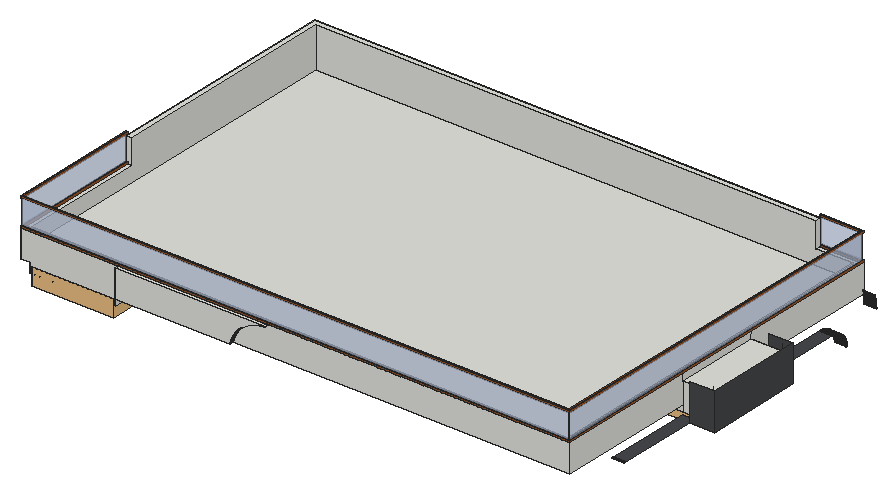
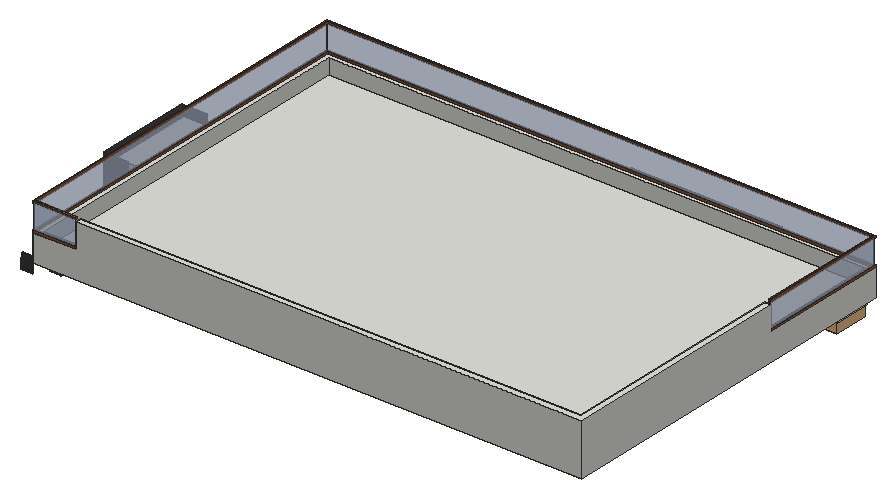
# SketchUp Ruby script. Lengths in inches.
U = 1.inch
M = Sketchup.active_model
def pt(a) = Geom::Point3d.new(a.map { |v| v * U })
def face(e, loops, mat)
  f = e.add_face(loops[0].map { |a| pt(a) })
  loops[1..].each { |l| e.add_face(l.map { |a| pt(a) }).erase! }
  f.material = f.back_material = mat if mat
  f
end
# faces: each face lists its corners as indices into pts; further lists are holes
def faces(e, pts, list, mat = nil) = list.each { |f| face(e, (f[0].is_a?(Array) ? f : [f]).map { |l| l.map { |i| pts[i] } }, mat) }
# xy, xz, yz: faces in a plane at the given z, y or x. An outline is a flat list of corners, or four numbers for a rectangle; further outlines are holes
def ring(l) = l.size == 4 ? [[l[0], l[1]], [l[2], l[1]], [l[2], l[3]], [l[0], l[3]]] : l.each_slice(2).to_a
def flat(e, list, mat, &to3) = list.each { |f| face(e, (f[0].is_a?(Array) ? f : [f]).map { |l| ring(l).map { |u, v| to3.(u, v) } }, mat) }
def xy(e, z, list, mat = nil) = flat(e, list, mat) { |x, y| [x, y, z] }
def xz(e, y, list, mat = nil) = flat(e, list, mat) { |x, z| [x, y, z] }
def yz(e, x, list, mat = nil) = flat(e, list, mat) { |y, z| [x, y, z] }
def lines(e, pts, list) = list.each { |a, b| e.add_line(pt(pts[a]), pt(pts[b])) }
# prism: a flat outline (further loops are holes) pulled along v
def prism(e, loops, v, mat = nil)
  f = face(e, loops, mat); d = Geom::Vector3d.new(v.map { |x| x * U })
  f.pushpull(f.normal.samedirection?(d) ? d.length : -d.length)
end
def box(e, o, s, mat = nil) = prism(e, [[o, [o[0] + s[0], o[1], o[2]], [o[0] + s[0], o[1] + s[1], o[2]], [o[0], o[1] + s[1], o[2]]]], [0, 0, s[2]], mat)
def at(x, y, z, deg = 0) = Geom::Transformation.translation(pt([x, y, z])) * Geom::Transformation.rotation(ORIGIN, Z_AXIS, deg.degrees)
def axes(o, x, y, z) = Geom::Transformation.new([*x, 0, *y, 0, *z, 0, *pt(o).to_a, 1])
def part(name) = M.definitions.add(name)
# library, detail: a bought-in or finely detailed component or shape, given as its bounding box
def library(name, o, s) = part(name).tap { |d| box(d.entities, o, s) }
def detail(e, o, s) = box(e.add_group.entities, o, s)
def put(e, d, t, mat = nil) = e.add_instance(d, t).tap { |i| i.material = mat if mat }
def group(e, t, mat = nil) = e.add_group.tap { |g| g.transformation = t; g.material = mat if mat }.entities
root = M.entities
M.materials.add("1432 AP 8245 TAR ROAD").color = [71, 72, 75]
M.materials.add("[Translucent Glass Blue]").color = [195, 208, 233]
M.materials["[Translucent Glass Blue]"].alpha = 0.5
M.materials.add("[Wood Cherry Original]").color = [152, 86, 42]
c1 = library("Group\#32",[0,0,-17.09],[62,80,17.09])
xy(root,560.79,[[573,160.9,585,161.13],[573,161.13,585,161.37],[573,161.37,573,245.37,603,245.37,603,329.37,573,329.37,573,413.37,585,413.37,585,335.37,609,335.37,609,239.37,585,239.37,585,161.37],[573,413.37,585,413.61],[573,413.61,585,413.84]],"1432 AP 8245 TAR ROAD")
xz(root,239.37,[[585,560.79,609,596.79]],"1432 AP 8245 TAR ROAD")
xz(root,335.37,[[585,560.79,609,596.79]],"1432 AP 8245 TAR ROAD")
xz(root,431.36,[[573,543.26,585,543.5]],"1432 AP 8245 TAR ROAD")
xz(root,431.37,[[573,542.79,585,543.03]],"1432 AP 8245 TAR ROAD")
xz(root,467.37,[[573,560.79,585,561.07],[573,561.07,585,561.36]],"1432 AP 8245 TAR ROAD")
yz(root,609,[[239.37,560.79,335.37,596.79]],"1432 AP 8245 TAR ROAD")
p = [[573,431.36,543.26],[573,431.37,543.03],[585,431.37,543.03],[585,431.36,543.26],[573,431.35,543.73],[573,431.36,543.5],
  [585,431.36,543.5],[585,431.35,543.73],[573,431.33,543.97],[585,431.33,543.97],[573,431.3125,544.2],[585,431.3125,544.2],
  [573,431.29,544.4375],[585,431.29,544.4375],[573,431.27,544.67],[585,431.27,544.67],[573,431.25,544.91],[585,431.25,544.91],
  [573,431.22,545.14],[585,431.22,545.14],[573,431.18,545.375],[585,431.18,545.375],[573,431.15,545.61],[585,431.15,545.61],
  [573,431.11,545.84],[585,431.11,545.84],[573,431.07,546.07],[585,431.07,546.07],[573,431.02,546.3],[585,431.02,546.3],
  [573,430.98,546.53],[585,430.98,546.53],[573,430.93,546.76],[585,430.93,546.76],[573,430.87,546.99],[585,430.87,546.99],
  [573,430.82,547.22],[585,430.82,547.22],[573,430.76,547.45],[585,430.76,547.45],[573,430.69,547.68],[585,430.69,547.68],
  [573,430.63,547.9],[585,430.63,547.9],[573,430.56,548.13],[585,430.56,548.13],[573,430.49,548.35],[585,430.49,548.35],
  [573,430.41,548.58],[585,430.41,548.58],[573,430.34,548.8],[585,430.34,548.8],[573,430.26,549.02],[585,430.26,549.02],
  [573,430.17,549.24],[585,430.17,549.24],[573,430.09,549.46],[585,430.09,549.46],[573,430,549.68],[585,430,549.68],
  [573,429.91,549.9],[585,429.91,549.9],[573,429.8125,550.11],[585,429.8125,550.11],[573,429.72,550.33],[585,429.72,550.33],
  [573,429.62,550.54],[585,429.62,550.54],[573,429.51,550.75],[585,429.51,550.75],[573,429.41,550.96],[585,429.41,550.96],
  [573,429.3,551.17],[585,429.3,551.17],[573,429.1875,551.38],[585,429.1875,551.38],[573,429.07,551.59],[585,429.07,551.59],
  [573,428.96,551.79],[585,428.96,551.79],[573,428.84,552],[585,428.84,552],[573,428.72,552.2],[585,428.72,552.2],
  [573,428.59,552.4],[585,428.59,552.4],[573,428.47,552.6],[585,428.47,552.6],[573,428.34,552.79],[585,428.34,552.79],
  [573,428.2,552.99],[585,428.2,552.99],[573,428.07,553.18],[585,428.07,553.18],[573,427.93,553.37],[585,427.93,553.37],
  [573,427.79,553.5625],[585,427.79,553.5625],[573,427.65,553.75],[585,427.65,553.75],[573,427.51,553.9375],[585,427.51,553.9375],
  [573,427.36,554.12],[585,427.36,554.12],[573,427.21,554.3],[585,427.21,554.3],[573,427.06,554.48],[585,427.06,554.48],
  [573,426.9,554.66],[585,426.9,554.66],[573,426.75,554.84],[585,426.75,554.84],[573,426.59,555.01],[585,426.59,555.01],
  [573,426.43,555.18],[585,426.43,555.18],[573,426.26,555.35],[585,426.26,555.35],[573,426.1,555.52],[585,426.1,555.52],
  [573,425.93,555.69],[585,425.93,555.69],[573,425.76,555.85],[585,425.76,555.85],[573,425.59,556.01],[585,425.59,556.01],
  [573,425.41,556.17],[585,425.41,556.17],[573,425.24,556.33],[585,425.24,556.33],[573,425.06,556.48],[585,425.06,556.48],
  [573,424.88,556.63],[585,424.88,556.63],[573,424.7,556.78],[585,424.7,556.78],[573,424.51,556.93],[585,424.51,556.93],
  [573,424.33,557.07],[585,424.33,557.07],[573,424.14,557.21],[585,424.14,557.21],[573,423.95,557.35],[585,423.95,557.35],
  [573,423.76,557.49],[585,423.76,557.49],[573,423.57,557.625],[585,423.57,557.625],[573,423.37,557.76],[585,423.37,557.76],
  [573,423.17,557.89],[585,423.17,557.89],[573,422.97,558.02],[585,422.97,558.02],[573,422.77,558.14],[585,422.77,558.14],
  [573,422.57,558.26],[585,422.57,558.26],[573,422.37,558.38],[585,422.37,558.38],[573,422.17,558.5],[585,422.17,558.5],
  [573,421.96,558.61],[585,421.96,558.61],[573,421.75,558.72],[585,421.75,558.72],[573,421.54,558.83],[585,421.54,558.83],
  [573,421.33,558.9375],[585,421.33,558.9375],[573,421.12,559.04],[585,421.12,559.04],[573,420.91,559.14],[585,420.91,559.14],
  [573,420.69,559.24],[585,420.69,559.24],[573,420.48,559.33],[585,420.48,559.33],[573,420.26,559.42],[585,420.26,559.42],
  [573,420.04,559.51],[585,420.04,559.51],[573,419.82,559.6],[585,419.82,559.6],[573,419.6,559.68],[585,419.6,559.68],
  [573,419.38,559.76],[585,419.38,559.76],[573,418.93,559.91],[573,419.16,559.84],[585,419.16,559.84],[585,418.93,559.91],
  [573,418.71,559.98],[585,418.71,559.98],[573,418.48,560.05],[585,418.48,560.05],[573,418.03,560.18],[573,418.26,560.12],
  [585,418.26,560.12],[585,418.03,560.18],[573,417.57,560.29],[573,417.8,560.24],[585,417.8,560.24],[585,417.57,560.29],
  [573,417.11,560.4],[573,417.34,560.35],[585,417.34,560.35],[585,417.11,560.4],[573,416.65,560.49],[573,416.88,560.45],
  [585,416.88,560.45],[585,416.65,560.49],[573,416.1875,560.57],[573,416.42,560.53],[585,416.42,560.53],[585,416.1875,560.57],
  [573,415.49,560.67],[573,415.72,560.64],[585,415.72,560.64],[585,415.49,560.67],[573,415.95,560.61],[585,415.95,560.61],
  [573,159.25,560.67],[573,159.49,560.69],[585,159.49,560.69],[585,159.25,560.67],[573,159.72,560.72],[585,159.72,560.72],
  [573,159.96,560.74],[585,159.96,560.74],[573,160.19,560.75],[585,160.19,560.75],[573,414.55,560.75],[573,414.78,560.74],
  [585,414.78,560.74],[585,414.55,560.75],[573,415.02,560.72],[585,415.02,560.72],[573,415.25,560.69],[585,415.25,560.69],
  [573,160.43,560.77],[585,160.43,560.77],[573,160.66,560.78],[585,160.66,560.78],[573,160.9,560.79],[585,160.9,560.79],
  [573,413.84,560.79],[573,414.08,560.78],[585,414.08,560.78],[585,413.84,560.79],[573,414.3125,560.77],[585,414.3125,560.77],
  [573,467.37,561.36],[573,467.36,561.64],[585,467.36,561.64],[585,467.37,561.36],[573,467.35,561.92],[585,467.35,561.92],
  [573,467.34,562.21],[585,467.34,562.21],[573,467.33,562.49],[585,467.33,562.49],[573,467.32,562.77],[585,467.32,562.77],
  [573,467.3,563.05],[585,467.3,563.05],[573,467.28,563.33],[585,467.28,563.33],[573,467.26,563.62],[585,467.26,563.62],
  [573,467.24,563.9],[585,467.24,563.9],[573,467.21,564.18],[585,467.21,564.18],[573,467.18,564.46],[585,467.18,564.46],
  [573,467.15,564.74],[585,467.15,564.74],[573,467.12,565.02],[585,467.12,565.02],[573,467.09,565.3],[585,467.09,565.3],
  [573,467.05,565.58],[585,467.05,565.58],[573,467.01,565.86],[585,467.01,565.86],[573,466.97,566.14],[585,466.97,566.14],
  [573,466.93,566.42],[585,466.93,566.42],[573,466.88,566.7],[585,466.88,566.7],[573,466.83,566.98],[585,466.83,566.98],
  [573,466.78,567.26],[585,466.78,567.26],[573,466.73,567.54],[585,466.73,567.54],[573,466.68,567.82],[585,466.68,567.82],
  [573,466.62,568.09],[585,466.62,568.09],[573,466.5625,568.37],[585,466.5625,568.37],[573,466.5,568.65],[585,466.5,568.65],
  [573,466.44,568.92],[585,466.44,568.92],[573,466.375,569.2],[585,466.375,569.2],[573,466.31,569.47],[585,466.31,569.47],
  [573,466.24,569.74],[585,466.24,569.74],[573,466.17,570.02],[585,466.17,570.02],[573,466.09,570.29],[585,466.09,570.29],
  [573,466.02,570.5625],[585,466.02,570.5625],[573,465.94,570.84],[585,465.94,570.84],[573,465.86,571.11],[585,465.86,571.11],
  [573,465.78,571.38],[585,465.78,571.38],[573,465.69,571.65],[585,465.69,571.65],[573,465.61,571.92],[585,465.61,571.92],
  [573,465.52,572.19],[585,465.52,572.19],[573,465.43,572.45],[585,465.43,572.45],[573,465.34,572.72],[585,465.34,572.72],
  [573,465.24,572.99],[585,465.24,572.99],[573,465.14,573.25],[585,465.14,573.25],[573,465.05,573.52],[585,465.05,573.52],
  [573,464.94,573.78],[585,464.94,573.78],[573,464.84,574.04],[585,464.84,574.04],[573,464.74,574.31],[585,464.74,574.31],
  [603,245.37,596.79],[603,245.37,560.79],[603,329.37,596.79],[603,329.37,560.79]]
faces(root,p,[[0,1,2,3],[4,5,6,7],[8,4,7,9],[10,8,9,11],[12,10,11,13],[14,12,13,15],[16,14,15,17],[18,16,17,19],
  [20,18,19,21],[22,20,21,23],[24,22,23,25],[26,24,25,27],[28,26,27,29],[30,28,29,31],[32,30,31,33],[34,32,33,35],
  [36,34,35,37],[38,36,37,39],[40,38,39,41],[42,40,41,43],[44,42,43,45],[46,44,45,47],[48,46,47,49],[50,48,49,51],
  [52,50,51,53],[54,52,53,55],[56,54,55,57],[58,56,57,59],[60,58,59,61],[62,60,61,63],[64,62,63,65],[66,64,65,67],
  [68,66,67,69],[70,68,69,71],[72,70,71,73],[74,72,73,75],[76,74,75,77],[78,76,77,79],[80,78,79,81],[82,80,81,83],
  [84,82,83,85],[86,84,85,87],[88,86,87,89],[90,88,89,91],[92,90,91,93],[94,92,93,95],[96,94,95,97],[98,96,97,99],
  [100,98,99,101],[102,100,101,103],[104,102,103,105],[106,104,105,107],[108,106,107,109],[110,108,109,111],[112,110,111,113],[114,112,113,115],
  [116,114,115,117],[118,116,117,119],[120,118,119,121],[122,120,121,123],[124,122,123,125],[126,124,125,127],[128,126,127,129],[130,128,129,131],
  [132,130,131,133],[134,132,133,135],[136,134,135,137],[138,136,137,139],[140,138,139,141],[142,140,141,143],[144,142,143,145],[146,144,145,147],
  [148,146,147,149],[150,148,149,151],[152,150,151,153],[154,152,153,155],[156,154,155,157],[158,156,157,159],[160,158,159,161],[162,160,161,163],
  [164,162,163,165],[166,164,165,167],[168,166,167,169],[170,168,169,171],[172,170,171,173],[174,172,173,175],[176,174,175,177],[178,176,177,179],
  [180,178,179,181],[182,180,181,183],[184,182,183,185],[186,184,185,187],[188,189,190,191],[189,186,187,190],[192,188,191,193],[194,192,193,195],
  [196,197,198,199],[197,194,195,198],[200,201,202,203],[201,196,199,202],[204,205,206,207],[205,200,203,206],[208,209,210,211],[209,204,207,210],
  [212,213,214,215],[213,208,211,214],[216,217,218,219],[217,220,221,218],[220,212,215,221],[222,223,224,225],[223,226,227,224],[226,228,229,227],
  [228,230,231,229],[232,233,234,235],[233,236,237,234],[236,238,239,237],[238,216,219,239],[230,240,241,231],[240,242,243,241],[242,244,245,243],
  [246,247,248,249],[247,250,251,248],[250,232,235,251],[252,253,254,255],[253,256,257,254],[256,258,259,257],[258,260,261,259],[260,262,263,261],
  [262,264,265,263],[264,266,267,265],[266,268,269,267],[268,270,271,269],[270,272,273,271],[272,274,275,273],[274,276,277,275],[276,278,279,277],
  [278,280,281,279],[280,282,283,281],[282,284,285,283],[284,286,287,285],[286,288,289,287],[288,290,291,289],[290,292,293,291],[292,294,295,293],
  [294,296,297,295],[296,298,299,297],[298,300,301,299],[300,302,303,301],[302,304,305,303],[304,306,307,305],[306,308,309,307],[308,310,311,309],
  [310,312,313,311],[312,314,315,313],[314,316,317,315],[316,318,319,317],[318,320,321,319],[320,322,323,321],[322,324,325,323],[324,326,327,325],
  [326,328,329,327],[328,330,331,329],[330,332,333,331],[332,334,335,333],[334,336,337,335],[336,338,339,337],[338,340,341,339],[340,342,343,341],
  [342,344,345,343],[344,346,347,345]],"1432 AP 8245 TAR ROAD")
lines(root,p,[[348,349],[350,351]])
g1 = group(root,at(45,116.37,569.79))
xy(g1,-9,[[[0,-8.9375,84,27],[2,-6.9375,82,25]]])
xy(g1,-6,[[[492,129,558,213],[494,131,556,211]]])
xy(g1,-3,[[2,-6.9375,82,25]])
xy(g1,0,[[87,-13,87,-8.9375,84,-8.9375,84,27,0,27,0,-8.9375,-9,-8.9375,-9,351,528,351,528,213,492,213,492,129,528,129,528,-9,199.14,-9,199.14,-13]])
xy(g1,2,[[494,131,556,211]])
xy(g1,12,[[-3,-3,522,345]])
xy(g1,21,[[528,129,558,213]])
xy(g1,27,[[87,-13,234,-13,234,-9,528,-9,528,351,486,351,486,345,522,345,522,-3,-3,-3,-3,120.0625,-9,120.0625,-9,-8.9375,87,-8.9375],[233.6,-13,234,-9]])
xy(g1,51,[[-9,120.0625,-3,120.0625,-3,345,486,345,486,351,-9,351]])
xz(g1,-13,[[87,0,199.14,0,199.25,0.38,199.35,0.76,199.46,1.14,199.58,1.52,199.69,1.9,199.82,2.27,199.94,2.65,200.07,3.02,200.49,4.13,200.64,4.5,200.79,4.86,200.94,5.23,201.1,5.59,201.27,5.95,201.43,6.31,201.6,6.66,201.78,7.02,202.14,7.72,202.52,8.42,202.71,8.76,203.11,9.44,203.3125,9.78,203.52,10.12,203.73,10.45,204.17,11.11,204.39,11.43,204.62,11.76,205.08,12.4,205.32,12.71,205.56,13.03,205.8,13.34,206.05,13.65,206.3,13.95,206.56,14.26,206.8125,14.56,207.07,14.85,207.34,15.15,207.61,15.4375,207.875,15.73,208.15,16.01,208.99,16.85,209.27,17.12,209.5625,17.39,209.85,17.66,210.75,18.44,211.35,18.94,211.97,19.44,212.29,19.68,212.6,19.91,212.92,20.15,213.24,20.375,213.57,20.6,213.9,20.82,214.22,21.04,214.56,21.26,215.22,21.68,215.5625,21.88,215.9,22.09,216.25,22.28,216.59,22.48,216.9375,22.67,217.29,22.85,218.34,23.39,218.7,23.56,219.06,23.72,219.42,23.89,219.78,24.04,220.14,24.2,220.88,24.5,221.62,24.78,222.36,25.04,222.74,25.17,223.11,25.29,223.49,25.41,224.25,25.63,224.625,25.74,225.01,25.84,225.39,25.9375,225.78,26.03,226.16,26.12,226.55,26.2,226.93,26.28,227.32,26.36,228.1,26.5,228.49,26.5625,228.88,26.62,229.27,26.68,229.66,26.73,230.06,26.77,230.45,26.82,230.84,26.85,231.24,26.89,231.63,26.92,232.03,26.94,232.81,26.98,233.21,26.99,233.6,27,234,27,87,27]])
xz(g1,-9,[[199.14,0,528,0,528,27,233.6,27,233.21,26.99,232.81,26.98,232.03,26.94,231.63,26.92,231.24,26.89,230.84,26.85,230.45,26.82,230.06,26.77,229.66,26.73,229.27,26.68,228.88,26.62,228.49,26.5625,228.1,26.5,227.32,26.36,226.93,26.28,226.55,26.2,226.16,26.12,225.78,26.03,225.39,25.9375,225.01,25.84,224.625,25.74,224.25,25.63,223.49,25.41,223.11,25.29,222.74,25.17,222.36,25.04,221.62,24.78,220.88,24.5,220.14,24.2,219.78,24.04,219.42,23.89,219.06,23.72,218.7,23.56,218.34,23.39,217.29,22.85,216.9375,22.67,216.59,22.48,216.25,22.28,215.9,22.09,215.5625,21.88,215.22,21.68,214.56,21.26,214.22,21.04,213.9,20.82,213.57,20.6,213.24,20.375,212.92,20.15,212.6,19.91,212.29,19.68,211.97,19.44,211.35,18.94,210.75,18.44,209.85,17.66,209.5625,17.39,209.27,17.12,208.99,16.85,208.15,16.01,207.875,15.73,207.61,15.4375,207.34,15.15,207.07,14.85,206.8125,14.56,206.56,14.26,206.3,13.95,206.05,13.65,205.8,13.34,205.56,13.03,205.32,12.71,205.08,12.4,204.62,11.76,204.39,11.43,204.17,11.11,203.73,10.45,203.52,10.12,203.3125,9.78,203.11,9.44,202.71,8.76,202.52,8.42,202.14,7.72,201.78,7.02,201.6,6.66,201.43,6.31,201.27,5.95,201.1,5.59,200.94,5.23,200.79,4.86,200.64,4.5,200.49,4.13,200.07,3.02,199.94,2.65,199.82,2.27,199.69,1.9,199.58,1.52,199.46,1.14,199.35,0.76,199.25,0.38]])
xz(g1,-8.9375,[[0,-9,84,-9,84,0,87,0,87,27,-9,27,-9,0,0,0]])
xz(g1,-6.9375,[[2,-9,82,-3]])
xz(g1,-3,[[-3,12,522,27]])
xz(g1,25,[[2,-9,82,-3]])
xz(g1,27,[[0,-9,84,0]])
xz(g1,120.0625,[[-9,27,-3,51]])
xz(g1,129,[[492,-6,528,0],[528,-6,558,21]])
xz(g1,131,[[494,-6,528,2],[528,-6,556,2]])
xz(g1,211,[[494,-6,528,2],[528,-6,556,2]])
xz(g1,213,[[492,-6,528,0],[528,-6,558,21]])
xz(g1,345,[[-3,12,522,12,522,27,486,27,486,51,-3,51]])
xz(g1,351,[[-9,0,-9,51,486,51,486,27,528,27,528,0]])
yz(g1,-9,[[-8.9375,0,-8.9375,27,120.0625,27,120.0625,51,351,51,351,0]])
yz(g1,-3,[[-3,12,345,12,345,51,120.0625,51,120.0625,27,-3,27]])
yz(g1,0,[[-8.9375,-9,27,0]])
yz(g1,2,[[-6.9375,-9,25,-3]])
yz(g1,82,[[-6.9375,-9,25,-3]])
yz(g1,84,[[-8.9375,-9,27,0]])
yz(g1,87,[[-13,0,-8.9375,27]])
yz(g1,486,[[345,27,351,51]])
yz(g1,492,[[129,-6,213,0]])
yz(g1,494,[[131,-6,211,2]])
yz(g1,522,[[-3,12,345,27]])
yz(g1,528,[[-9,0,129,27],[213,0,351,27],[129,21,213,27]])
yz(g1,556,[[131,-6,211,2]])
yz(g1,558,[[129,-6,213,21]])
p = [[199.25,-13,0.38],[199.14,-13,0],[199.14,-9,0],[199.25,-9,0.38],[199.35,-13,0.76],[199.35,-9,0.76],
  [199.46,-13,1.14],[199.46,-9,1.14],[199.58,-13,1.52],[199.58,-9,1.52],[199.69,-13,1.9],[199.69,-9,1.9],
  [199.82,-13,2.27],[199.82,-9,2.27],[199.94,-13,2.65],[199.94,-9,2.65],[200.07,-13,3.02],[200.07,-9,3.02],
  [200.21,-13,3.39],[200.21,-9,3.39],[200.35,-13,3.76],[200.35,-9,3.76],[200.49,-13,4.13],[200.49,-9,4.13],
  [200.64,-13,4.5],[200.64,-9,4.5],[200.79,-13,4.86],[200.79,-9,4.86],[200.94,-13,5.23],[200.94,-9,5.23],
  [201.1,-13,5.59],[201.1,-9,5.59],[201.27,-13,5.95],[201.27,-9,5.95],[201.43,-13,6.31],[201.43,-9,6.31],
  [201.6,-13,6.66],[201.6,-9,6.66],[201.78,-13,7.02],[201.78,-9,7.02],[201.96,-13,7.37],[201.96,-9,7.37],
  [202.14,-13,7.72],[202.14,-9,7.72],[202.33,-13,8.07],[202.33,-9,8.07],[202.52,-13,8.42],[202.52,-9,8.42],
  [202.71,-13,8.76],[202.71,-9,8.76],[202.91,-13,9.1],[202.91,-9,9.1],[203.11,-13,9.44],[203.11,-9,9.44],
  [203.3125,-13,9.78],[203.3125,-9,9.78],[203.52,-13,10.12],[203.52,-9,10.12],[203.73,-13,10.45],[203.73,-9,10.45],
  [203.95,-13,10.78],[203.95,-9,10.78],[204.17,-13,11.11],[204.17,-9,11.11],[204.39,-13,11.43],[204.39,-9,11.43],
  [204.62,-13,11.76],[204.62,-9,11.76],[204.85,-13,12.08],[204.85,-9,12.08],[205.08,-13,12.4],[205.08,-9,12.4],
  [205.32,-13,12.71],[205.32,-9,12.71],[205.56,-13,13.03],[205.56,-9,13.03],[205.8,-13,13.34],[205.8,-9,13.34],
  [206.05,-13,13.65],[206.05,-9,13.65],[206.3,-13,13.95],[206.3,-9,13.95],[206.56,-13,14.26],[206.56,-9,14.26],
  [206.8125,-13,14.56],[206.8125,-9,14.56],[207.07,-13,14.85],[207.07,-9,14.85],[207.34,-13,15.15],[207.34,-9,15.15],
  [207.61,-13,15.4375],[207.61,-9,15.4375],[207.875,-13,15.73],[207.875,-9,15.73],[208.15,-13,16.01],[208.15,-9,16.01],
  [208.43,-13,16.29],[208.43,-9,16.29],[208.71,-13,16.57],[208.71,-9,16.57],[208.99,-13,16.85],[208.99,-9,16.85],
  [209.27,-13,17.12],[209.27,-9,17.12],[209.5625,-13,17.39],[209.5625,-9,17.39],[209.85,-13,17.66],[209.85,-9,17.66],
  [210.15,-13,17.92],[210.15,-9,17.92],[210.45,-13,18.18],[210.45,-9,18.18],[210.75,-13,18.44],[210.75,-9,18.44],
  [211.05,-13,18.69],[211.05,-9,18.69],[211.35,-13,18.94],[211.35,-9,18.94],[211.66,-13,19.19],[211.66,-9,19.19],
  [211.97,-13,19.44],[211.97,-9,19.44],[212.29,-13,19.68],[212.29,-9,19.68],[212.6,-13,19.91],[212.6,-9,19.91],
  [212.92,-13,20.15],[212.92,-9,20.15],[213.24,-13,20.375],[213.24,-9,20.375],[213.57,-13,20.6],[213.57,-9,20.6],
  [213.9,-13,20.82],[213.9,-9,20.82],[214.22,-13,21.04],[214.22,-9,21.04],[214.56,-13,21.26],[214.56,-9,21.26],
  [214.89,-13,21.47],[214.89,-9,21.47],[215.22,-13,21.68],[215.22,-9,21.68],[215.5625,-13,21.88],[215.5625,-9,21.88],
  [215.9,-13,22.09],[215.9,-9,22.09],[216.25,-13,22.28],[216.25,-9,22.28],[216.59,-13,22.48],[216.59,-9,22.48],
  [216.9375,-13,22.67],[216.9375,-9,22.67],[217.29,-13,22.85],[217.29,-9,22.85],[217.64,-13,23.03],[217.64,-9,23.03],
  [217.99,-13,23.21],[217.99,-9,23.21],[218.34,-13,23.39],[218.34,-9,23.39],[218.7,-13,23.56],[218.7,-9,23.56],
  [219.06,-13,23.72],[219.06,-9,23.72],[219.42,-13,23.89],[219.42,-9,23.89],[219.78,-13,24.04],[219.78,-9,24.04],
  [220.14,-13,24.2],[220.14,-9,24.2],[220.51,-13,24.35],[220.51,-9,24.35],[220.88,-13,24.5],[220.88,-9,24.5],
  [221.25,-13,24.64],[221.25,-9,24.64],[221.62,-13,24.78],[221.62,-9,24.78],[221.99,-13,24.91],[221.99,-9,24.91],
  [222.36,-13,25.04],[222.36,-9,25.04],[222.74,-13,25.17],[222.74,-9,25.17],[223.11,-13,25.29],[223.11,-9,25.29],
  [223.49,-13,25.41],[223.49,-9,25.41],[223.87,-13,25.52],[223.87,-9,25.52],[224.25,-13,25.63],[224.25,-9,25.63],
  [224.625,-13,25.74],[224.625,-9,25.74],[225.01,-13,25.84],[225.01,-9,25.84],[225.39,-13,25.9375],[225.39,-9,25.9375],
  [225.78,-13,26.03],[225.78,-9,26.03],[226.16,-13,26.12],[226.16,-9,26.12],[226.55,-13,26.2],[226.55,-9,26.2],
  [226.93,-13,26.28],[226.93,-9,26.28],[227.32,-13,26.36],[227.32,-9,26.36],[227.71,-13,26.43],[227.71,-9,26.43],
  [228.1,-13,26.5],[228.1,-9,26.5],[228.49,-13,26.5625],[228.49,-9,26.5625],[228.88,-13,26.62],[228.88,-9,26.62],
  [229.27,-13,26.68],[229.27,-9,26.68],[229.66,-13,26.73],[229.66,-9,26.73],[230.06,-13,26.77],[230.06,-9,26.77],
  [230.45,-13,26.82],[230.45,-9,26.82],[230.84,-13,26.85],[230.84,-9,26.85],[231.24,-13,26.89],[231.24,-9,26.89],
  [231.63,-13,26.92],[231.63,-9,26.92],[232.03,-13,26.94],[232.03,-9,26.94],[232.42,-13,26.96],[232.42,-9,26.96],
  [232.81,-13,26.98],[232.81,-9,26.98],[233.21,-13,26.99],[233.21,-9,26.99],[233.6,-13,27],[233.6,-9,27],
  [199.28,-9,0.5],[199.36,-9,0.8],[199.45,-9,1.1],[199.54,-9,1.4],[199.63,-9,1.7],[199.72,-9,2],
  [199.82,-9,2.3],[199.92,-9,2.59],[200.02,-9,2.89],[200.125,-9,3.18],[200.23,-9,3.48],[200.34,-9,3.77],
  [200.45,-9,4.0625],[200.57,-9,4.35],[200.6875,-9,4.64],[200.81,-9,4.93],[200.93,-9,5.22],[201.05,-9,5.51],
  [201.18,-9,5.79],[201.31,-9,6.08],[201.44,-9,6.36],[201.58,-9,6.64],[201.71,-9,6.93],[201.85,-9,7.21],
  [202,-9,7.48],[202.14,-9,7.76],[202.29,-9,8.04],[202.4375,-9,8.3125],[202.59,-9,8.59],[202.74,-9,8.86],
  [202.9,-9,9.13],[203.06,-9,9.4],[203.22,-9,9.67],[203.38,-9,9.94],[203.55,-9,10.2],[203.72,-9,10.46],
  [203.89,-9,10.73],[204.06,-9,10.99],[204.23,-9,11.25],[204.41,-9,11.51],[204.59,-9,11.76],[204.77,-9,12.02],
  [204.96,-9,12.27],[205.14,-9,12.52],[205.33,-9,12.77],[205.52,-9,13.02],[205.71,-9,13.27],[205.91,-9,13.51],
  [206.1,-9,13.76],[206.3,-9,14],[206.5,-9,14.24],[206.71,-9,14.47],[206.91,-9,14.71],[207.12,-9,14.95],
  [207.33,-9,15.18],[207.54,-9,15.41],[207.75,-9,15.64],[207.97,-9,15.87],[208.18,-9,16.09],[208.4,-9,16.3125],
  [208.625,-9,16.54],[208.85,-9,16.76],[209.07,-9,16.97],[209.3,-9,17.1875],[209.53,-9,17.4],[209.76,-9,17.61],
  [209.99,-9,17.82],[210.22,-9,18.03],[210.46,-9,18.24],[210.7,-9,18.44],[210.9375,-9,18.64],[211.18,-9,18.84],
  [211.42,-9,19.04],[211.67,-9,19.23],[211.91,-9,19.43],[212.16,-9,19.62],[212.41,-9,19.81],[212.66,-9,19.99],
  [212.91,-9,20.18],[213.17,-9,20.36],[213.42,-9,20.54],[213.68,-9,20.72],[213.94,-9,20.89],[214.2,-9,21.07],
  [214.46,-9,21.24],[214.73,-9,21.41],[214.99,-9,21.57],[215.26,-9,21.74],[215.53,-9,21.9],[215.79,-9,22.06],
  [216.07,-9,22.21],[216.34,-9,22.37],[216.61,-9,22.52],[216.89,-9,22.67],[217.16,-9,22.82],[217.4375,-9,22.96],
  [217.72,-9,23.11],[218,-9,23.25],[218.28,-9,23.39],[218.56,-9,23.52],[218.84,-9,23.65],[219.13,-9,23.78],
  [219.41,-9,23.91],[219.7,-9,24.04],[219.99,-9,24.16],[220.28,-9,24.28],[220.57,-9,24.4],[220.86,-9,24.51],
  [221.15,-9,24.63],[221.44,-9,24.74],[221.73,-9,24.85],[222.03,-9,24.95],[222.32,-9,25.05],[222.62,-9,25.15],
  [222.92,-9,25.25],[223.22,-9,25.35],[223.52,-9,25.4375],[223.82,-9,25.53],[224.12,-9,25.62],[224.42,-9,25.7],
  [224.72,-9,25.78],[225.02,-9,25.86],[225.32,-9,25.9375],[225.63,-9,26.01],[225.93,-9,26.08],[226.24,-9,26.15],
  [226.54,-9,26.22],[226.85,-9,26.28],[227.16,-9,26.34],[227.47,-9,26.4],[227.77,-9,26.46],[228.08,-9,26.51],
  [228.39,-9,26.56],[228.7,-9,26.61],[229.01,-9,26.65],[229.32,-9,26.69],[229.63,-9,26.73],[229.94,-9,26.77],
  [230.25,-9,26.8],[230.5625,-9,26.84],[230.875,-9,26.86],[231.1875,-9,26.89],[231.5,-9,26.91],[231.8125,-9,26.93],
  [232.125,-9,26.95],[232.4375,-9,26.97],[232.75,-9,26.98],[233.0625,-9,26.99],[233.375,-9,26.99],[233.6875,-9,27],
  [234,-9,27]]
faces(g1,p,[[0,1,2,3],[4,0,3,5],[6,4,5,7],[8,6,7,9],[10,8,9,11],[12,10,11,13],[14,12,13,15],[16,14,15,17],
  [18,16,17,19],[20,18,19,21],[22,20,21,23],[24,22,23,25],[26,24,25,27],[28,26,27,29],[30,28,29,31],[32,30,31,33],
  [34,32,33,35],[36,34,35,37],[38,36,37,39],[40,38,39,41],[42,40,41,43],[44,42,43,45],[46,44,45,47],[48,46,47,49],
  [50,48,49,51],[52,50,51,53],[54,52,53,55],[56,54,55,57],[58,56,57,59],[60,58,59,61],[62,60,61,63],[64,62,63,65],
  [66,64,65,67],[68,66,67,69],[70,68,69,71],[72,70,71,73],[74,72,73,75],[76,74,75,77],[78,76,77,79],[80,78,79,81],
  [82,80,81,83],[84,82,83,85],[86,84,85,87],[88,86,87,89],[90,88,89,91],[92,90,91,93],[94,92,93,95],[96,94,95,97],
  [98,96,97,99],[100,98,99,101],[102,100,101,103],[104,102,103,105],[106,104,105,107],[108,106,107,109],[110,108,109,111],[112,110,111,113],
  [114,112,113,115],[116,114,115,117],[118,116,117,119],[120,118,119,121],[122,120,121,123],[124,122,123,125],[126,124,125,127],[128,126,127,129],
  [130,128,129,131],[132,130,131,133],[134,132,133,135],[136,134,135,137],[138,136,137,139],[140,138,139,141],[142,140,141,143],[144,142,143,145],
  [146,144,145,147],[148,146,147,149],[150,148,149,151],[152,150,151,153],[154,152,153,155],[156,154,155,157],[158,156,157,159],[160,158,159,161],
  [162,160,161,163],[164,162,163,165],[166,164,165,167],[168,166,167,169],[170,168,169,171],[172,170,171,173],[174,172,173,175],[176,174,175,177],
  [178,176,177,179],[180,178,179,181],[182,180,181,183],[184,182,183,185],[186,184,185,187],[188,186,187,189],[190,188,189,191],[192,190,191,193],
  [194,192,193,195],[196,194,195,197],[198,196,197,199],[200,198,199,201],[202,200,201,203],[204,202,203,205],[206,204,205,207],[208,206,207,209],
  [210,208,209,211],[212,210,211,213],[214,212,213,215],[216,214,215,217],[218,216,217,219],[220,218,219,221],[222,220,221,223],[224,222,223,225],
  [226,224,225,227],[228,226,227,229],[230,228,229,231],[232,230,231,233],[234,232,233,235],[236,234,235,237],[238,236,237,239]])
lines(g1,p,[[240,241],[241,242],[242,243],[243,244],[244,245],[245,246],[246,247],[247,248],[248,249],[249,250],[250,251],[251,252],
  [252,253],[253,254],[254,255],[255,256],[256,257],[257,258],[258,259],[259,260],[260,261],[261,262],[262,263],[263,264],
  [264,265],[265,266],[266,267],[267,268],[268,269],[269,270],[270,271],[271,272],[272,273],[273,274],[274,275],[275,276],
  [276,277],[277,278],[278,279],[279,280],[280,281],[281,282],[282,283],[283,284],[284,285],[285,286],[286,287],[287,288],
  [288,289],[289,290],[290,291],[291,292],[292,293],[293,294],[294,295],[295,296],[296,297],[297,298],[298,299],[299,300],
  [300,301],[301,302],[302,303],[303,304],[304,305],[305,306],[306,307],[307,308],[308,309],[309,310],[310,311],[311,312],
  [312,313],[313,314],[314,315],[315,316],[316,317],[317,318],[318,319],[319,320],[320,321],[321,322],[322,323],[323,324],
  [324,325],[325,326],[326,327],[327,328],[328,329],[329,330],[330,331],[331,332],[332,333],[333,334],[334,335],[335,336],
  [336,337],[337,338],[338,339],[339,340],[340,341],[341,342],[342,343],[343,344],[344,345],[345,346],[346,347],[347,348],
  [348,349],[349,350],[350,351],[351,352],[352,353],[353,354],[354,355],[355,356],[356,357],[357,358],[358,359],[359,360],
  [360,361],[361,362],[362,363],[363,364],[364,365],[365,366],[366,367],[367,368],[368,369],[369,370],[370,371],[371,372],
  [372,373],[373,374],[374,375],[375,376],[376,377],[377,378],[378,379],[379,380],[380,381],[381,382],[382,383],[383,384],
  [384,385],[385,386],[386,387],[387,388],[388,239],[389,390],[239,389]])
put(g1,c1,at(494,131,2))
g2 = group(g1,at(-9,-9,27),"[Wood Cherry Original]")
xy(g2,0,[[0,0,0,129.0625,2,129.0625,2,2,535,2,535,358,495,358,495,360,537,360,537,0]])
xy(g2,1.5,[[0.75,0.75,536.25,0.75,536.25,359.25,495.75,359.25,495.75,358.75,535.75,358.75,535.75,1.25,1.25,1.25,1.25,128.3125,0.75,128.3125]])
xy(g2,2,[[[0,0,537,0,537,360,495,360,495,358,535,358,535,2,2,2,2,129.0625,0,129.0625],[0.75,0.75,0.75,128.3125,1.25,128.3125,1.25,1.25,535.75,1.25,535.75,358.75,495.75,358.75,495.75,359.25,536.25,359.25,536.25,0.75]]])
xy(g2,26,[[[0,0,0,129.0625,2,129.0625,2,2,535,2,535,358,495,358,495,360,537,360,537,0],[0.75,0.75,536.25,0.75,536.25,359.25,495.75,359.25,495.75,358.75,535.75,358.75,535.75,1.25,1.25,1.25,1.25,128.3125,0.75,128.3125]]])
xy(g2,26.5,[[0.75,0.75,0.75,128.3125,1.25,128.3125,1.25,1.25,535.75,1.25,535.75,358.75,495.75,358.75,495.75,359.25,536.25,359.25,536.25,0.75]])
xy(g2,28,[[0,0,537,0,537,360,495,360,495,358,535,358,535,2,2,2,2,129.0625,0,129.0625]])
xz(g2,0,[[0,0,537,2],[0,26,537,28]])
xz(g2,0.75,[[0.75,1.5,536.25,2],[0.75,26,536.25,26.5]])
xz(g2,1.25,[[1.25,1.5,535.75,2],[1.25,26,535.75,26.5]])
xz(g2,2,[[2,0,535,2],[2,26,535,28]])
xz(g2,128.3125,[[0.75,1.5,1.25,2],[0.75,26,1.25,26.5]])
xz(g2,129.0625,[[0,0,2,2],[0,26,2,28]])
xz(g2,358,[[495,0,535,2],[495,26,535,28]])
xz(g2,358.75,[[495.75,1.5,535.75,2],[495.75,26,535.75,26.5]])
xz(g2,359.25,[[495.75,1.5,536.25,2],[495.75,26,536.25,26.5]])
xz(g2,360,[[495,0,537,2],[495,26,537,28]])
yz(g2,0,[[0,0,129.0625,2],[0,26,129.0625,28]])
yz(g2,0.75,[[0.75,1.5,128.3125,2],[0.75,26,128.3125,26.5]])
yz(g2,1.25,[[1.25,1.5,128.3125,2],[1.25,26,128.3125,26.5]])
yz(g2,2,[[2,0,129.0625,2],[2,26,129.0625,28]])
yz(g2,495,[[358,0,360,2],[358,26,360,28]])
yz(g2,495.75,[[358.75,1.5,359.25,2],[358.75,26,359.25,26.5]])
yz(g2,535,[[2,0,358,2],[2,26,358,28]])
yz(g2,535.75,[[1.25,1.5,358.75,2],[1.25,26,358.75,26.5]])
yz(g2,536.25,[[0.75,1.5,359.25,2],[0.75,26,359.25,26.5]])
yz(g2,537,[[0,0,360,2],[0,26,360,28]])
g3 = group(g2,at(0.75,0.75,1.5),"[Translucent Glass Blue]")
prism(g3,[[[0,0,0],[0,127.5625,0],[0.5,127.5625,0],[0.5,0.5,0],[535,0.5,0],[535,358,0],[495,358,0],[495,358.5,0],[535.5,358.5,0],[535.5,0,0]]],[0,0,25])
put(g1,c1,axes([2,25,-3],[0,-0.54839,0],[1,0,0],[0,0,1]))
